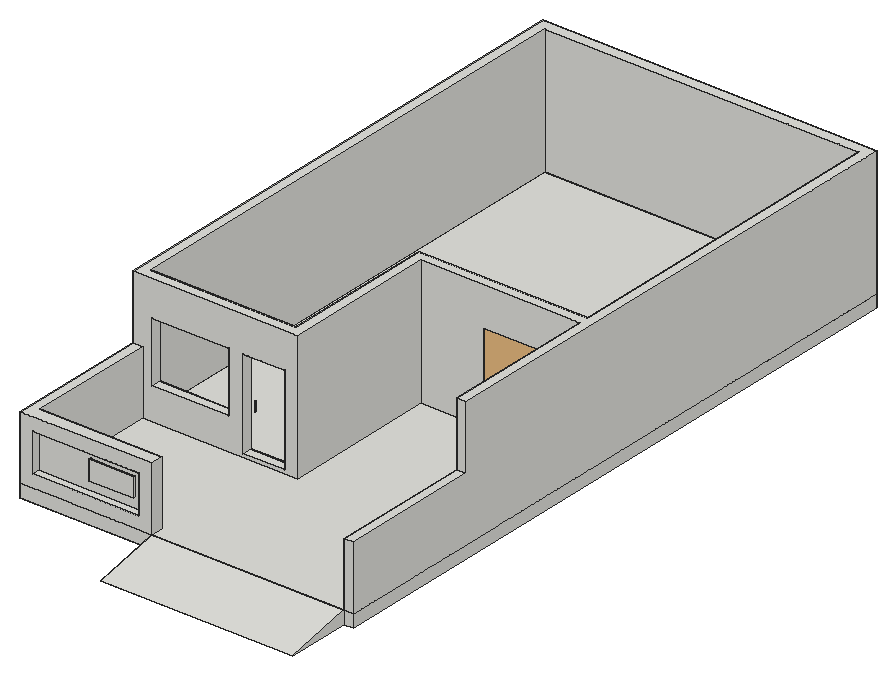
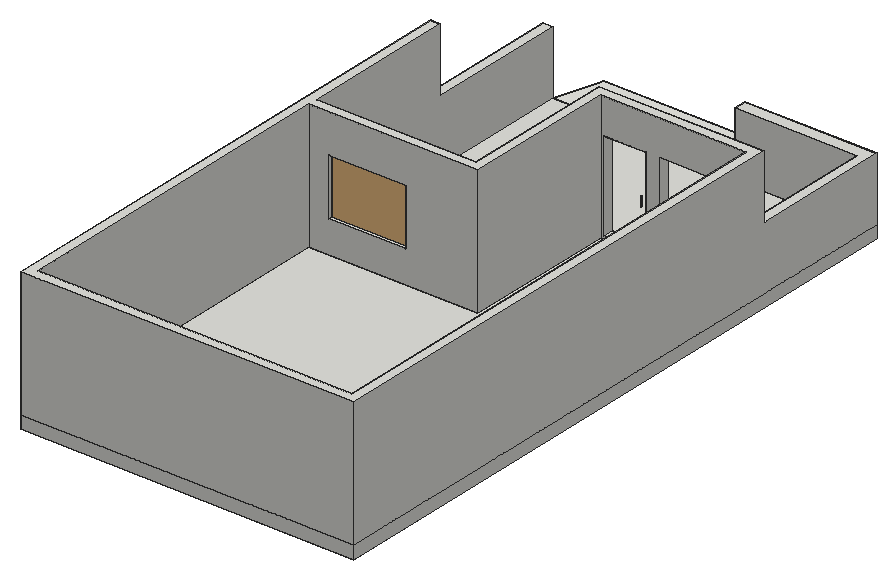
# SketchUp Ruby script. Lengths in inches.
U = 1.inch
M = Sketchup.active_model
def pt(a) = Geom::Point3d.new(a.map { |v| v * U })
def face(e, loops, mat)
  f = e.add_face(loops[0].map { |a| pt(a) })
  loops[1..].each { |l| e.add_face(l.map { |a| pt(a) }).erase! }
  f.material = f.back_material = mat if mat
  f
end
# faces: each face lists its corners as indices into pts; further lists are holes
def faces(e, pts, list, mat = nil) = list.each { |f| face(e, (f[0].is_a?(Array) ? f : [f]).map { |l| l.map { |i| pts[i] } }, mat) }
# xy, xz, yz: faces in a plane at the given z, y or x. An outline is a flat list of corners, or four numbers for a rectangle; further outlines are holes
def ring(l) = l.size == 4 ? [[l[0], l[1]], [l[2], l[1]], [l[2], l[3]], [l[0], l[3]]] : l.each_slice(2).to_a
def flat(e, list, mat, &to3) = list.each { |f| face(e, (f[0].is_a?(Array) ? f : [f]).map { |l| ring(l).map { |u, v| to3.(u, v) } }, mat) }
def xy(e, z, list, mat = nil) = flat(e, list, mat) { |x, y| [x, y, z] }
def xz(e, y, list, mat = nil) = flat(e, list, mat) { |x, z| [x, y, z] }
def yz(e, x, list, mat = nil) = flat(e, list, mat) { |y, z| [x, y, z] }
def lines(e, pts, list) = list.each { |a, b| e.add_line(pt(pts[a]), pt(pts[b])) }
# prism: a flat outline (further loops are holes) pulled along v
def prism(e, loops, v, mat = nil)
  f = face(e, loops, mat); d = Geom::Vector3d.new(v.map { |x| x * U })
  f.pushpull(f.normal.samedirection?(d) ? d.length : -d.length)
end
def box(e, o, s, mat = nil) = prism(e, [[o, [o[0] + s[0], o[1], o[2]], [o[0] + s[0], o[1] + s[1], o[2]], [o[0], o[1] + s[1], o[2]]]], [0, 0, s[2]], mat)
def at(x, y, z, deg = 0) = Geom::Transformation.translation(pt([x, y, z])) * Geom::Transformation.rotation(ORIGIN, Z_AXIS, deg.degrees)
def axes(o, x, y, z) = Geom::Transformation.new([*x, 0, *y, 0, *z, 0, *pt(o).to_a, 1])
def part(name) = M.definitions.add(name)
# library, detail: a bought-in or finely detailed component or shape, given as its bounding box
def library(name, o, s) = part(name).tap { |d| box(d.entities, o, s) }
def detail(e, o, s) = box(e.add_group.entities, o, s)
def put(e, d, t, mat = nil) = e.add_instance(d, t).tap { |i| i.material = mat if mat }
def group(e, t, mat = nil) = e.add_group.tap { |g| g.transformation = t; g.material = mat if mat }.entities
root = M.entities
M.materials.add("Material \#1").color = [140, 140, 140]
c1 = library("Multi-panel window",[0,0,0],[5.02,84.63,60])
xy(root,0,[[[0,60,0,672,312,672,312,72,303,72,303,336,154.049,336,154.049,192,9,192,9,72,123,72,123,60],[9,201,145.049,201,145.049,345,303,345,303,663,9,663]],[303,60,312,72]])
xy(root,3,[[103.049,192,142.049,201]])
xy(root,12,[[12,60,111,67]])
xy(root,21,[[60,65,102,67]])
xy(root,30,[[18,192,90,201],[213,336,285,345]])
xy(root,39,[[60,65,102,67]])
xy(root,48,[[12,60,111,67]])
xy(root,60,[[0,60,123,60,123,72,9,72,9,192,0,192],[303,60,312,192]])
xy(root,84,[[213,336,285,345]])
xy(root,87,[[18,192,90,201],[103.049,192,142.049,201]])
xy(root,120,[[[0,192,154.049,192,154.049,336,303,336,303,192,312,192,312,672,0,672],[9,201,9,663,303,663,303,345,145.049,345,145.049,201]]])
xz(root,60,[[[0,0,123,60],[12,12,111,48]],[303,0,312,60]])
xz(root,65,[[60,21,102,39]])
xz(root,67,[[[12,12,111,48],[60,21,102,39]]])
xz(root,72,[[9,0,123,60]])
xz(root,192,[[[9,0,154.049,0,154.049,120,0,120,0,60,9,60],[18,30,90,87],[103.049,3,142.049,87]],[303,60,312,120]])
xz(root,198.681,[[109.188,37.641,109.188,37.652,109.3,37.663],[109.188,37.641,109.3,37.663,109.302,37.652],[108.968,37.684,108.869,37.734,108.972,37.695],[108.972,37.695,108.869,37.734,108.875,37.745],[108.869,37.734,108.781,37.802,108.875,37.745],
  [108.875,37.745,108.781,37.802,108.788,37.811],[109.595,37.802,109.588,37.811,109.663,37.893],[109.595,37.802,109.663,37.893,109.671,37.885],[109.188,37.824,109.151,37.828,109.188,37.836],[109.188,37.824,109.188,37.836,109.224,37.84],
  [109.188,37.824,109.224,37.84,109.226,37.828],[109.151,37.828,109.115,37.839,109.152,37.84],[109.151,37.828,109.152,37.84,109.188,37.836],[109.115,37.839,109.119,37.85,109.152,37.84],[109.294,37.855,109.288,37.866,109.316,37.887],
  [109.294,37.855,109.316,37.887,109.323,37.878],[109.323,37.878,109.316,37.887,109.34,37.913],[109.323,37.878,109.34,37.913,109.348,37.905],[109.348,37.905,109.34,37.913,109.36,37.943],[109.348,37.905,109.36,37.943,109.369,37.937],
  [109.369,37.937,109.36,37.943,109.375,37.977],[109.369,37.937,109.375,37.977,109.385,37.973],[109.385,37.973,109.375,37.977,109.384,38.014],[109.385,37.973,109.384,38.014,109.395,38.012],[109.395,38.012,109.384,38.014,109.387,38.052],
  [109.395,38.012,109.387,38.052,109.398,38.052],[109.387,38.052,109.384,38.091,109.398,38.052],[109.398,38.052,109.384,38.091,109.395,38.093],[109.384,38.091,109.375,38.128,109.395,38.093],[109.395,38.093,109.375,38.128,109.385,38.132],
  [109.375,38.128,109.36,38.161,109.385,38.132],[109.385,38.132,109.36,38.161,109.369,38.167],[109.36,38.161,109.34,38.192,109.369,38.167],[109.369,38.167,109.34,38.192,109.348,38.199],[109.34,38.192,109.316,38.218,109.348,38.199],
  [109.348,38.199,109.316,38.218,109.323,38.227],[109.809,38.204,109.799,38.206,109.809,38.332],[109.809,38.204,109.809,38.332,109.82,38.331],[109.316,38.218,109.288,38.239,109.323,38.227],[109.323,38.227,109.288,38.239,109.294,38.249],
  [109.288,38.239,109.257,38.255,109.294,38.249],[109.294,38.249,109.257,38.255,109.261,38.266],[109.257,38.255,109.224,38.265,109.261,38.266],[109.152,38.265,109.188,38.28,109.188,38.269],[109.224,38.265,109.188,38.269,109.226,38.277],
  [109.224,38.265,109.226,38.277,109.261,38.266],[109.188,38.269,109.188,38.28,109.226,38.277],[108.556,38.331,108.556,46.173,108.567,38.332],[109.82,38.331,109.809,38.332,109.809,44.483],[109.82,38.331,109.809,44.483,109.809,46.173],
  [109.82,38.331,109.809,46.173,109.82,46.173],[108.567,38.332,108.556,46.173,108.567,46.173],[108.556,46.173,108.567,46.301,108.567,46.173],[108.567,46.173,108.567,46.301,108.577,46.299],[109.809,46.173,109.799,46.299,109.82,46.173],
  [109.82,46.173,109.799,46.299,109.809,46.301],[109.188,46.224,109.151,46.228,109.188,46.236],[109.188,46.224,109.188,46.236,109.224,46.24],[109.188,46.224,109.224,46.24,109.226,46.228],[109.151,46.228,109.115,46.239,109.152,46.24],
  [109.151,46.228,109.152,46.24,109.188,46.236],[109.226,46.228,109.224,46.24,109.257,46.25],[109.226,46.228,109.257,46.25,109.261,46.239],[109.115,46.239,109.082,46.255,109.119,46.25],[109.115,46.239,109.119,46.25,109.152,46.24],
  [109.261,46.239,109.257,46.25,109.288,46.266],[109.261,46.239,109.288,46.266,109.294,46.255],[109.119,46.25,109.082,46.255,109.088,46.266],[109.082,46.255,109.053,46.278,109.088,46.266],[109.294,46.255,109.288,46.266,109.316,46.287],
  [109.294,46.255,109.316,46.287,109.323,46.278],[109.088,46.266,109.053,46.278,109.06,46.287],[109.053,46.278,109.028,46.305,109.06,46.287],[109.323,46.278,109.316,46.287,109.34,46.313],[109.323,46.278,109.34,46.313,109.348,46.305],
  [109.06,46.287,109.028,46.305,109.036,46.313],[108.577,46.299,108.567,46.301,108.596,46.417],[108.577,46.299,108.596,46.417,108.606,46.413],[109.799,46.299,109.77,46.413,109.809,46.301],[109.809,46.301,109.77,46.413,109.78,46.417],
  [109.028,46.305,109.007,46.337,109.036,46.313],[109.348,46.305,109.34,46.313,109.36,46.343],[109.348,46.305,109.36,46.343,109.369,46.337],[109.036,46.313,109.007,46.337,109.016,46.343],[109.007,46.337,108.991,46.373,109.016,46.343],
  [109.369,46.337,109.36,46.343,109.375,46.377],[109.369,46.337,109.375,46.377,109.385,46.373],[109.016,46.343,108.991,46.373,109.002,46.377],[108.991,46.373,108.982,46.412,109.002,46.377],[109.385,46.373,109.375,46.377,109.384,46.414],
  [109.385,46.373,109.384,46.414,109.395,46.412],[109.002,46.377,108.982,46.412,108.992,46.414],[108.982,46.412,108.978,46.463,108.992,46.414],[109.395,46.412,109.384,46.414,109.387,46.452],[109.395,46.412,109.387,46.452,109.398,46.452],
  [108.606,46.413,108.596,46.417,108.643,46.524],[108.606,46.413,108.643,46.524,108.652,46.518],[109.77,46.413,109.724,46.518,109.78,46.417],[108.992,46.414,108.978,46.463,108.989,46.463],[109.78,46.417,109.724,46.518,109.733,46.524],
  [109.387,46.452,109.384,46.491,109.398,46.452],[109.398,46.452,109.384,46.491,109.395,46.493],[108.978,46.463,108.982,46.493,108.989,46.463],[108.989,46.463,108.982,46.493,108.992,46.491],[108.992,46.491,108.982,46.493,108.991,46.532],
  [108.992,46.491,108.991,46.532,109.002,46.528],[109.384,46.491,109.375,46.528,109.395,46.493],[109.395,46.493,109.375,46.528,109.385,46.532],[108.652,46.518,108.643,46.524,108.708,46.623],[108.652,46.518,108.708,46.623,108.716,46.615],
  [109.724,46.518,109.663,46.612,109.733,46.524],[109.733,46.524,109.663,46.612,109.671,46.62],[109.002,46.528,108.991,46.532,109.007,46.567],[109.002,46.528,109.007,46.567,109.016,46.561],[109.375,46.528,109.36,46.561,109.385,46.532],
  [109.385,46.532,109.36,46.561,109.369,46.567],[109.016,46.561,109.007,46.567,109.028,46.599],[109.016,46.561,109.028,46.599,109.036,46.592],[109.36,46.561,109.34,46.592,109.369,46.567],[109.369,46.567,109.34,46.592,109.348,46.599],
  [109.036,46.592,109.028,46.599,109.053,46.627],[109.036,46.592,109.053,46.627,109.06,46.618],[109.34,46.592,109.316,46.618,109.348,46.599],[109.348,46.599,109.316,46.618,109.323,46.627],[109.663,46.612,109.588,46.694,109.671,46.62],
  [108.716,46.615,108.708,46.623,108.781,46.703],[108.716,46.615,108.781,46.703,108.788,46.693],[109.06,46.618,109.053,46.627,109.082,46.649],[109.06,46.618,109.082,46.649,109.088,46.639],[109.316,46.618,109.288,46.639,109.323,46.627],
  [109.671,46.62,109.588,46.694,109.595,46.703],[109.323,46.627,109.288,46.639,109.294,46.649],[109.088,46.639,109.082,46.649,109.115,46.666],[109.088,46.639,109.115,46.666,109.119,46.655],[109.288,46.639,109.257,46.655,109.294,46.649],
  [109.294,46.649,109.257,46.655,109.261,46.666],[109.119,46.655,109.115,46.666,109.151,46.677],[109.119,46.655,109.151,46.677,109.152,46.665],[109.257,46.655,109.224,46.665,109.261,46.666],[109.152,46.665,109.151,46.677,109.188,46.68],
  [109.152,46.665,109.188,46.68,109.188,46.669],[109.224,46.665,109.188,46.669,109.226,46.677],[109.224,46.665,109.226,46.677,109.261,46.666],[109.188,46.669,109.188,46.68,109.226,46.677],[108.788,46.693,108.781,46.703,108.869,46.77],
  [108.788,46.693,108.869,46.77,108.875,46.76],[109.588,46.694,109.501,46.76,109.595,46.703],[109.595,46.703,109.501,46.76,109.507,46.77],[108.875,46.76,108.869,46.77,108.968,46.821],[108.875,46.76,108.968,46.821,108.972,46.81],
  [109.501,46.76,109.405,46.81,109.507,46.77],[109.507,46.77,109.405,46.81,109.408,46.821],[108.972,46.81,108.968,46.821,109.074,46.853],[108.972,46.81,109.074,46.853,109.076,46.841],[109.405,46.81,109.3,46.841,109.408,46.821],
  [109.408,46.821,109.3,46.841,109.302,46.853],[109.076,46.841,109.074,46.853,109.188,46.864],[109.076,46.841,109.188,46.864,109.188,46.852],[109.3,46.841,109.188,46.852,109.302,46.853],[109.188,46.852,109.188,46.864,109.302,46.853]],"Material \#1")
xz(root,198.714,[[109.188,40.003,109.081,40.059,109.295,40.059],[109.188,40.003,109.128,40.018,109.081,40.059],[109.188,40.003,109.157,40.007,109.128,40.018],[109.188,40.003,109.248,40.018,109.22,40.007],[109.188,40.003,109.295,40.059,109.248,40.018],
  [109.128,40.018,109.102,40.036,109.081,40.059],[109.248,40.018,109.295,40.059,109.274,40.036],[109.295,40.059,108.945,40.647,109.019,40.535],[109.295,40.059,109.046,40.46,108.945,40.647],[109.295,40.059,109.019,40.535,109.053,40.498],
  [109.295,40.059,109.048,40.455,109.046,40.46],[109.295,40.059,109.05,40.45,109.048,40.455],[109.295,40.059,109.051,40.444,109.05,40.45],[109.081,40.059,109.051,40.438,109.051,40.444],[109.081,40.059,109.051,40.444,109.295,40.059],
  [109.081,40.059,109.054,40.118,109.051,40.438],[109.295,40.059,109.053,40.498,109.093,40.471],[109.081,40.059,109.065,40.087,109.054,40.118],[109.295,40.059,109.093,40.471,109.138,40.453],[109.295,40.059,109.138,40.453,109.188,40.447],
  [109.295,40.059,109.188,40.447,109.325,40.152],[109.295,40.059,109.322,40.118,109.311,40.087],[109.295,40.059,109.325,40.152,109.322,40.118],[109.054,40.118,109.051,40.152,109.051,40.438],[109.325,40.152,109.188,40.447,109.238,40.453],
  [109.325,40.152,109.238,40.453,109.283,40.471],[109.325,40.152,109.283,40.471,109.324,40.498],[109.325,40.152,109.324,40.498,109.325,40.4375],[109.325,40.4375,109.324,40.498,109.327,40.45],[109.325,40.4375,109.327,40.45,109.326,40.444],
  [109.327,40.45,109.324,40.498,109.357,40.535],[109.327,40.45,109.331,40.461,109.328,40.456],[109.327,40.45,109.357,40.535,109.331,40.461],[109.046,40.46,109.042,40.466,108.945,40.647],[109.331,40.461,109.357,40.535,109.383,40.579],
  [109.331,40.461,109.383,40.579,109.431,40.647],[109.331,40.461,109.431,40.647,109.334,40.466],[109.042,40.466,109.039,40.47,108.945,40.647],[109.334,40.466,109.431,40.647,109.338,40.47],[109.039,40.47,108.991,40.523,108.945,40.647],
  [109.039,40.47,109.034,40.475,108.991,40.523],[109.338,40.47,109.384,40.524,109.342,40.475],[109.338,40.47,109.431,40.647,109.384,40.524],[109.034,40.475,109.011,40.497,108.991,40.523],[109.342,40.475,109.384,40.524,109.364,40.498],
  [108.991,40.523,108.961,40.581,108.945,40.647],[108.991,40.523,108.975,40.551,108.961,40.581],[109.384,40.524,109.415,40.581,109.401,40.551],[109.384,40.524,109.431,40.647,109.415,40.581],[109.019,40.535,108.945,40.647,108.993,40.579],
  [108.993,40.579,108.945,40.647,108.977,40.628],[109.383,40.579,109.399,40.628,109.431,40.647],[108.961,40.581,108.951,40.613,108.945,40.647],[109.415,40.581,109.431,40.647,109.425,40.613],[108.977,40.628,108.945,40.647,108.971,40.682],
  [109.399,40.628,109.405,40.682,109.431,40.647],[108.945,40.647,108.943,40.682,108.949,40.743],[108.945,40.647,108.949,40.743,108.996,40.849],[108.945,40.647,108.977,40.736,108.971,40.682],[108.945,40.647,108.996,40.849,108.977,40.736],
  [109.431,40.647,109.38,40.849,109.427,40.743],[109.431,40.647,109.383,40.786,109.38,40.849],[109.431,40.647,109.399,40.736,109.383,40.786],[109.431,40.647,109.405,40.682,109.399,40.736],[109.431,40.647,109.427,40.743,109.434,40.682],
  [108.977,40.736,108.996,40.849,108.993,40.786],[108.949,40.743,108.967,40.8,108.996,40.849],[109.427,40.743,109.38,40.849,109.409,40.8],[108.993,40.786,108.996,40.849,109.019,40.829],[109.383,40.786,109.357,40.829,109.38,40.849],
  [109.019,40.829,108.996,40.849,109.053,40.866],[109.357,40.829,109.324,40.866,109.38,40.849],[108.996,40.849,109.035,40.89,109.08,40.922],[108.996,40.849,109.08,40.922,109.188,40.949],[108.996,40.849,109.093,40.894,109.053,40.866],
  [108.996,40.849,109.188,40.949,109.093,40.894],[109.38,40.849,109.188,40.949,109.296,40.922],[109.38,40.849,109.283,40.894,109.188,40.949],[109.38,40.849,109.324,40.866,109.283,40.894],[109.38,40.849,109.296,40.922,109.342,40.89],
  [109.093,40.894,109.188,40.949,109.138,40.912],[109.283,40.894,109.238,40.912,109.188,40.949],[109.138,40.912,109.188,40.949,109.188,40.918],[109.238,40.912,109.188,40.918,109.188,40.949],[109.08,40.922,109.132,40.942,109.188,40.949],
  [109.296,40.922,109.188,40.949,109.244,40.942]],"Material \#1")
xz(root,198.724,[[109.188,40.472,109.138,40.479,109.188,40.48],[109.188,40.472,109.188,40.48,109.236,40.487],[109.188,40.472,109.236,40.487,109.238,40.479],[109.138,40.479,109.092,40.5,109.14,40.487],[109.138,40.479,109.14,40.487,109.188,40.48],
  [109.238,40.479,109.236,40.487,109.281,40.507],[109.238,40.479,109.281,40.507,109.285,40.5],[109.14,40.487,109.092,40.5,109.095,40.507],[109.092,40.5,109.052,40.534,109.095,40.507],[109.285,40.5,109.281,40.507,109.319,40.539],
  [109.285,40.5,109.319,40.539,109.325,40.534],[109.095,40.507,109.052,40.534,109.057,40.539],[109.052,40.534,109.021,40.577,109.057,40.539],[109.325,40.534,109.319,40.539,109.349,40.581],[109.325,40.534,109.349,40.581,109.355,40.577],
  [109.057,40.539,109.021,40.577,109.027,40.581],[109.021,40.577,109.002,40.628,109.027,40.581],[109.355,40.577,109.349,40.581,109.368,40.63],[109.355,40.577,109.368,40.63,109.375,40.628],[109.027,40.581,109.002,40.628,109.009,40.63],
  [109.002,40.628,108.995,40.682,109.009,40.63],[109.375,40.628,109.368,40.63,109.374,40.682],[109.375,40.628,109.374,40.682,109.381,40.682],[109.009,40.63,108.995,40.682,109.002,40.682],[108.995,40.682,109.002,40.737,109.002,40.682],
  [109.002,40.682,109.002,40.737,109.009,40.735],[109.374,40.682,109.368,40.735,109.381,40.682],[109.381,40.682,109.368,40.735,109.375,40.737],[109.009,40.735,109.002,40.737,109.021,40.787],[109.009,40.735,109.021,40.787,109.027,40.783],
  [109.368,40.735,109.349,40.783,109.375,40.737],[109.375,40.737,109.349,40.783,109.355,40.787],[109.027,40.783,109.021,40.787,109.052,40.831],[109.027,40.783,109.052,40.831,109.057,40.825],[109.349,40.783,109.319,40.825,109.355,40.787],
  [109.355,40.787,109.319,40.825,109.325,40.831],[109.057,40.825,109.052,40.831,109.092,40.864],[109.057,40.825,109.092,40.864,109.095,40.857],[109.319,40.825,109.281,40.857,109.325,40.831],[109.325,40.831,109.281,40.857,109.285,40.864],
  [109.095,40.857,109.092,40.864,109.138,40.885],[109.095,40.857,109.138,40.885,109.14,40.877],[109.281,40.857,109.236,40.877,109.285,40.864],[109.285,40.864,109.236,40.877,109.238,40.885],[109.14,40.877,109.138,40.885,109.188,40.892],
  [109.14,40.877,109.188,40.892,109.188,40.884],[109.236,40.877,109.188,40.884,109.238,40.885],[109.188,40.884,109.188,40.892,109.238,40.885]],"Material \#1")
xz(root,201,[[[9,0,145.049,120],[18,30,90,87],[103.049,3,142.049,87]]])
xz(root,336,[[[154.049,0,303,120],[213,30,285,84]]])
xz(root,345,[[[145.049,0,303,120],[213,30,285,84]]])
xz(root,663,[[9,0,303,120]])
xz(root,672,[[0,0,312,120]])
yz(root,0,[[60,0,60,60,192,60,192,120,672,120,672,0]])
yz(root,9,[[72,0,192,60],[201,0,663,120]])
yz(root,12,[[60,12,67,48]])
yz(root,18,[[192,30,201,87]])
yz(root,60,[[65,21,67,39]])
yz(root,90,[[192,30,201,87]])
yz(root,102,[[65,21,67,39]])
yz(root,103.049,[[192,3,201,87]])
yz(root,111,[[60,12,67,48]])
yz(root,123,[[60,0,72,60]])
yz(root,142.049,[[192,3,201,87]])
yz(root,145.049,[[201,0,345,120]])
yz(root,154.049,[[192,0,336,120]])
yz(root,213,[[336,30,345,84]])
yz(root,285,[[336,30,345,84]])
yz(root,303,[[60,0,60,60,192,60,192,120,336,120,336,0],[345,0,663,120]])
yz(root,312,[[60,0,672,0,672,120,192,120,192,60,60,60]])
p = [[303,336,0],[303,345,0]]
lines(root,p,[[0,1]])
g1 = group(root,at(9,201,0))
xy(g1,-12,[[-9,-141,303,471]])
xy(g1,0,[[-9,-141,303,471]])
xz(g1,-141,[[-9,-12,114,0],[294,-12,303,0]])
xz(g1,471,[[-9,-12,303,0]])
yz(g1,-9,[[-141,-12,471,0]])
yz(g1,303,[[-141,-12,471,0]])
g2 = group(g1,at(114,-141,-12))
prism(g2,[[[180,0,0],[180,0,12],[180,-60,0]]],[-180,0,0])
put(root,c1,axes([213,341.02,30],[0,-0.84,0],[0.85075,0,0],[0,0,0.9]))
